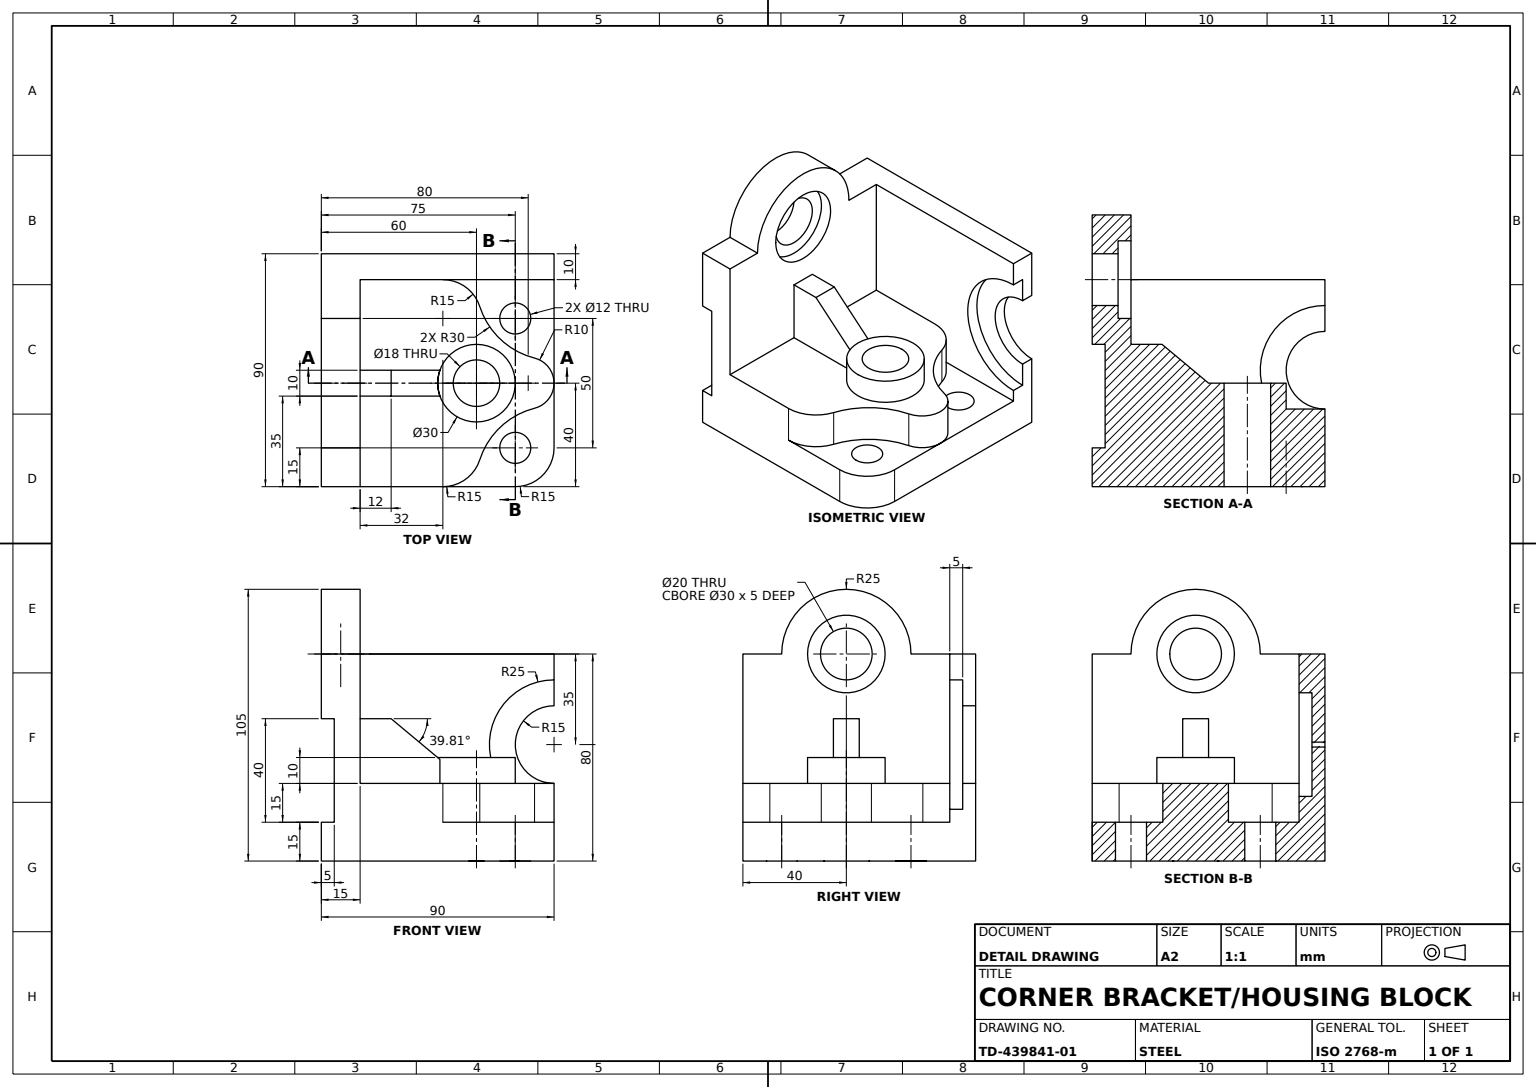
ISO-10303-21;
HEADER;
FILE_DESCRIPTION((''),'2;1');
FILE_NAME('','',(''),(''),'','','');
FILE_SCHEMA(('AUTOMOTIVE_DESIGN'));
ENDSEC;
DATA;
#1=APPLICATION_CONTEXT('');
#2=PRODUCT_CONTEXT('',#1,'mechanical');
#3=PRODUCT('','','',(#2));
#4=PRODUCT_DEFINITION_FORMATION('','',#3);
#5=PRODUCT_DEFINITION_CONTEXT('',#1,'design');
#6=PRODUCT_DEFINITION('','',#4,#5);
#7=PRODUCT_DEFINITION_SHAPE('','',#6);
#8=(LENGTH_UNIT()NAMED_UNIT(*)SI_UNIT(.MILLI.,.METRE.));
#9=(NAMED_UNIT(*)PLANE_ANGLE_UNIT()SI_UNIT($,.RADIAN.));
#10=(NAMED_UNIT(*)SI_UNIT($,.STERADIAN.)SOLID_ANGLE_UNIT());
#11=UNCERTAINTY_MEASURE_WITH_UNIT(LENGTH_MEASURE(1.E-05),#8,'distance_accuracy_value','');
#12=(GEOMETRIC_REPRESENTATION_CONTEXT(3)GLOBAL_UNCERTAINTY_ASSIGNED_CONTEXT((#11))GLOBAL_UNIT_ASSIGNED_CONTEXT((#8,#9,#10))REPRESENTATION_CONTEXT('',''));
#13=CARTESIAN_POINT('',(30.,-0.000006,-19.));
#14=VERTEX_POINT('',#13);
#15=CARTESIAN_POINT('',(30.,15.,-19.));
#16=VERTEX_POINT('',#15);
#17=CARTESIAN_POINT('',(30.,-0.000012,-19.));
#18=DIRECTION('',(0.,1.,0.));
#19=VECTOR('',#18,1000.);
#20=LINE('',#17,#19);
#21=EDGE_CURVE('',#14,#16,#20,.T.);
#22=ORIENTED_EDGE('',*,*,#21,.F.);
#23=CARTESIAN_POINT('',(30.,-0.000006,-31.));
#24=VERTEX_POINT('',#23);
#25=CARTESIAN_POINT('',(29.214602,-0.000012,-19.));
#26=CARTESIAN_POINT('',(28.429513,-0.000012,-19.156164));
#27=CARTESIAN_POINT('',(26.978286,-0.000012,-19.757282));
#28=CARTESIAN_POINT('',(26.31272,-0.000012,-20.201999));
#29=CARTESIAN_POINT('',(25.201999,-0.000012,-21.31272));
#30=CARTESIAN_POINT('',(24.757282,-0.000012,-21.978286));
#31=CARTESIAN_POINT('',(24.156164,-0.000012,-23.429513));
#32=CARTESIAN_POINT('',(24.,-0.000012,-24.214602));
#33=CARTESIAN_POINT('',(24.,-0.000012,-25.785398));
#34=CARTESIAN_POINT('',(24.156164,-0.000012,-26.570487));
#35=CARTESIAN_POINT('',(24.757282,-0.000012,-28.021714));
#36=CARTESIAN_POINT('',(25.201999,-0.000012,-28.68728));
#37=CARTESIAN_POINT('',(26.31272,-0.000012,-29.798001));
#38=CARTESIAN_POINT('',(26.978286,-0.000012,-30.242718));
#39=CARTESIAN_POINT('',(28.429513,-0.000012,-30.843836));
#40=CARTESIAN_POINT('',(29.214602,-0.000012,-31.));
#41=B_SPLINE_CURVE_WITH_KNOTS('',3,(#13,#25,#26,#27,#28,#29,#30,#31,#32,#33,#34,#35,#36,#37,#38,#39,#40,#23),.UNSPECIFIED.,.F.,.F.,(4,2,2,2,2,2,2,2,4),(0.5,0.5625,0.625,0.6875,0.75,0.8125,0.875,0.9375,1.),.UNSPECIFIED.);
#42=EDGE_CURVE('',#14,#24,#41,.T.);
#43=ORIENTED_EDGE('',*,*,#42,.T.);
#44=CARTESIAN_POINT('',(30.,15.,-31.));
#45=VERTEX_POINT('',#44);
#46=CARTESIAN_POINT('',(30.,-0.000012,-31.));
#47=LINE('',#46,#19);
#48=EDGE_CURVE('',#24,#45,#47,.T.);
#49=ORIENTED_EDGE('',*,*,#48,.T.);
#50=CARTESIAN_POINT('',(30.,15.,-25.));
#51=DIRECTION('',(0.,0.,-1.));
#52=AXIS2_PLACEMENT_3D('',#50,#18,#51);
#53=CIRCLE('',#52,6.);
#54=EDGE_CURVE('',#45,#16,#53,.T.);
#55=ORIENTED_EDGE('',*,*,#54,.T.);
#56=EDGE_LOOP('',(#22,#43,#49,#55));
#57=FACE_OUTER_BOUND('',#56,.T.);
#58=CARTESIAN_POINT('',(30.,-0.000012,-25.));
#59=DIRECTION('',(0.,0.,1.));
#60=AXIS2_PLACEMENT_3D('',#58,#18,#59);
#61=CYLINDRICAL_SURFACE('',#60,6.);
#62=ADVANCED_FACE('',(#57),#61,.F.);
#63=CARTESIAN_POINT('',(-45.,80.,-10.));
#64=VERTEX_POINT('',#63);
#65=CARTESIAN_POINT('',(-45.,80.,10.));
#66=VERTEX_POINT('',#65);
#67=CARTESIAN_POINT('',(-45.,80.,0.));
#68=DIRECTION('',(-1.,0.,0.));
#69=AXIS2_PLACEMENT_3D('',#67,#68,#59);
#70=CIRCLE('',#69,10.);
#71=EDGE_CURVE('',#64,#66,#70,.T.);
#72=ORIENTED_EDGE('',*,*,#71,.T.);
#73=CARTESIAN_POINT('',(-35.,80.,10.));
#74=VERTEX_POINT('',#73);
#75=CARTESIAN_POINT('',(-30.,80.,10.));
#76=DIRECTION('',(1.,0.,0.));
#77=VECTOR('',#76,1000.);
#78=LINE('',#75,#77);
#79=EDGE_CURVE('',#66,#74,#78,.T.);
#80=ORIENTED_EDGE('',*,*,#79,.T.);
#81=CARTESIAN_POINT('',(-35.,80.,-10.));
#82=VERTEX_POINT('',#81);
#83=CARTESIAN_POINT('',(-35.,80.,0.));
#84=AXIS2_PLACEMENT_3D('',#83,#76,#51);
#85=CIRCLE('',#84,10.);
#86=EDGE_CURVE('',#74,#82,#85,.T.);
#87=ORIENTED_EDGE('',*,*,#86,.T.);
#88=CARTESIAN_POINT('',(-30.,80.,-10.));
#89=LINE('',#88,#77);
#90=EDGE_CURVE('',#64,#82,#89,.T.);
#91=ORIENTED_EDGE('',*,*,#90,.F.);
#92=EDGE_LOOP('',(#72,#80,#87,#91));
#93=FACE_OUTER_BOUND('',#92,.T.);
#94=CARTESIAN_POINT('',(-30.,80.,0.));
#95=AXIS2_PLACEMENT_3D('',#94,#76,#51);
#96=CYLINDRICAL_SURFACE('',#95,10.);
#97=ADVANCED_FACE('',(#93),#96,.F.);
#98=CARTESIAN_POINT('',(-45.,80.,-25.));
#99=VERTEX_POINT('',#98);
#100=CARTESIAN_POINT('',(-45.,80.,-50.));
#101=VERTEX_POINT('',#100);
#102=CARTESIAN_POINT('',(-45.,80.,-40.));
#103=VECTOR('',#51,1000.);
#104=LINE('',#102,#103);
#105=EDGE_CURVE('',#99,#101,#104,.T.);
#106=ORIENTED_EDGE('',*,*,#105,.F.);
#107=CARTESIAN_POINT('',(-30.,80.,-25.));
#108=VERTEX_POINT('',#107);
#109=VECTOR('',#68,1000.);
#110=LINE('',#107,#109);
#111=EDGE_CURVE('',#108,#99,#110,.T.);
#112=ORIENTED_EDGE('',*,*,#111,.F.);
#113=CARTESIAN_POINT('',(-30.,80.,-40.));
#114=VERTEX_POINT('',#113);
#115=CARTESIAN_POINT('',(-30.,80.,40.));
#116=LINE('',#115,#103);
#117=EDGE_CURVE('',#108,#114,#116,.T.);
#118=ORIENTED_EDGE('',*,*,#117,.T.);
#119=CARTESIAN_POINT('',(45.,80.,-40.));
#120=VERTEX_POINT('',#119);
#121=LINE('',#102,#77);
#122=EDGE_CURVE('',#114,#120,#121,.T.);
#123=ORIENTED_EDGE('',*,*,#122,.T.);
#124=CARTESIAN_POINT('',(45.,80.,-50.));
#125=VERTEX_POINT('',#124);
#126=LINE('',#119,#103);
#127=EDGE_CURVE('',#120,#125,#126,.T.);
#128=ORIENTED_EDGE('',*,*,#127,.T.);
#129=LINE('',#100,#77);
#130=EDGE_CURVE('',#101,#125,#129,.T.);
#131=ORIENTED_EDGE('',*,*,#130,.F.);
#132=EDGE_LOOP('',(#106,#112,#118,#123,#128,#131));
#133=FACE_OUTER_BOUND('',#132,.T.);
#134=AXIS2_PLACEMENT_3D('',#102,#18,#59);
#135=PLANE('',#134);
#136=ADVANCED_FACE('',(#133),#135,.T.);
#137=CARTESIAN_POINT('',(45.,15.,0.));
#138=VERTEX_POINT('',#137);
#139=CARTESIAN_POINT('',(37.460317,15.,-9.692618));
#140=VERTEX_POINT('',#139);
#141=CARTESIAN_POINT('',(35.,15.,0.));
#142=AXIS2_PLACEMENT_3D('',#141,#18,#51);
#143=CIRCLE('',#142,10.);
#144=EDGE_CURVE('',#138,#140,#143,.T.);
#145=ORIENTED_EDGE('',*,*,#144,.T.);
#146=CARTESIAN_POINT('',(37.460317,30.,-9.692618));
#147=VERTEX_POINT('',#146);
#148=DIRECTION('',(0.,-1.,0.));
#149=VECTOR('',#148,1000.);
#150=LINE('',#146,#149);
#151=EDGE_CURVE('',#147,#140,#150,.T.);
#152=ORIENTED_EDGE('',*,*,#151,.F.);
#153=CARTESIAN_POINT('',(37.460317,30.,9.692618));
#154=VERTEX_POINT('',#153);
#155=CARTESIAN_POINT('',(35.,30.,0.));
#156=AXIS2_PLACEMENT_3D('',#155,#18,#59);
#157=CIRCLE('',#156,10.);
#158=EDGE_CURVE('',#154,#147,#157,.T.);
#159=ORIENTED_EDGE('',*,*,#158,.F.);
#160=CARTESIAN_POINT('',(37.460317,15.,9.692618));
#161=VERTEX_POINT('',#160);
#162=LINE('',#153,#149);
#163=EDGE_CURVE('',#154,#161,#162,.T.);
#164=ORIENTED_EDGE('',*,*,#163,.T.);
#165=EDGE_CURVE('',#161,#138,#143,.T.);
#166=ORIENTED_EDGE('',*,*,#165,.T.);
#167=EDGE_LOOP('',(#145,#152,#159,#164,#166));
#168=FACE_OUTER_BOUND('',#167,.T.);
#169=AXIS2_PLACEMENT_3D('',#155,#148,#51);
#170=CYLINDRICAL_SURFACE('',#169,10.);
#171=ADVANCED_FACE('',(#168),#170,.T.);
#172=CARTESIAN_POINT('',(15.,-0.000006,-9.));
#173=VERTEX_POINT('',#172);
#174=CARTESIAN_POINT('',(15.,-0.000006,9.));
#175=VERTEX_POINT('',#174);
#176=CARTESIAN_POINT('',(13.806876,0.,-9.00007));
#177=CARTESIAN_POINT('',(12.658179,0.,-8.77144));
#178=CARTESIAN_POINT('',(10.453519,0.,-7.858391));
#179=CARTESIAN_POINT('',(9.479754,0.,-7.207578));
#180=CARTESIAN_POINT('',(7.792324,0.,-5.520344));
#181=CARTESIAN_POINT('',(7.141737,0.,-4.546427));
#182=CARTESIAN_POINT('',(6.228431,0.,-2.341874));
#183=CARTESIAN_POINT('',(6.00007,0.,-1.193124));
#184=CARTESIAN_POINT('',(5.99993,0.,1.193124));
#185=CARTESIAN_POINT('',(6.22856,0.,2.341821));
#186=CARTESIAN_POINT('',(7.141609,0.,4.546481));
#187=CARTESIAN_POINT('',(7.792422,0.,5.520246));
#188=CARTESIAN_POINT('',(9.479656,0.,7.207676));
#189=CARTESIAN_POINT('',(10.453405,0.,7.858193));
#190=CARTESIAN_POINT('',(12.658294,0.,8.771639));
#191=CARTESIAN_POINT('',(13.806344,0.,9.));
#192=B_SPLINE_CURVE_WITH_KNOTS('',3,(#172,#176,#177,#178,#179,#180,#181,#182,#183,#184,#185,#186,#187,#188,#189,#190,#191,#174),.UNSPECIFIED.,.F.,.F.,(4,2,2,2,2,2,2,2,4),(0.5,0.5625,0.625,0.6875,0.75,0.8125,0.875,0.9375,1.),.UNSPECIFIED.);
#193=EDGE_CURVE('',#173,#175,#192,.T.);
#194=ORIENTED_EDGE('',*,*,#193,.F.);
#195=CARTESIAN_POINT('',(15.,40.,-9.));
#196=VERTEX_POINT('',#195);
#197=LINE('',#195,#149);
#198=EDGE_CURVE('',#196,#173,#197,.T.);
#199=ORIENTED_EDGE('',*,*,#198,.F.);
#200=CARTESIAN_POINT('',(15.,40.,9.));
#201=VERTEX_POINT('',#200);
#202=CARTESIAN_POINT('',(15.,40.,0.));
#203=AXIS2_PLACEMENT_3D('',#202,#18,#59);
#204=CIRCLE('',#203,9.);
#205=EDGE_CURVE('',#196,#201,#204,.T.);
#206=ORIENTED_EDGE('',*,*,#205,.T.);
#207=LINE('',#200,#149);
#208=EDGE_CURVE('',#201,#175,#207,.T.);
#209=ORIENTED_EDGE('',*,*,#208,.T.);
#210=EDGE_LOOP('',(#194,#199,#206,#209));
#211=FACE_OUTER_BOUND('',#210,.T.);
#212=AXIS2_PLACEMENT_3D('',#202,#148,#51);
#213=CYLINDRICAL_SURFACE('',#212,9.);
#214=ADVANCED_FACE('',(#211),#213,.F.);
#215=CARTESIAN_POINT('',(-30.,30.,5.));
#216=VERTEX_POINT('',#215);
#217=CARTESIAN_POINT('',(-30.,55.,5.));
#218=VERTEX_POINT('',#217);
#219=CARTESIAN_POINT('',(-30.,80.,5.));
#220=LINE('',#219,#19);
#221=EDGE_CURVE('',#216,#218,#220,.T.);
#222=ORIENTED_EDGE('',*,*,#221,.F.);
#223=CARTESIAN_POINT('',(0.857864,30.,5.));
#224=VERTEX_POINT('',#223);
#225=CARTESIAN_POINT('',(35.,30.,5.));
#226=LINE('',#225,#77);
#227=EDGE_CURVE('',#216,#224,#226,.T.);
#228=ORIENTED_EDGE('',*,*,#227,.T.);
#229=CARTESIAN_POINT('',(0.857864,39.285113,5.));
#230=VERTEX_POINT('',#229);
#231=CARTESIAN_POINT('',(0.857864,40.,5.));
#232=LINE('',#231,#149);
#233=EDGE_CURVE('',#230,#224,#232,.T.);
#234=ORIENTED_EDGE('',*,*,#233,.F.);
#235=CARTESIAN_POINT('',(-18.,55.,5.));
#236=VERTEX_POINT('',#235);
#237=DIRECTION('',(0.76822128,-0.6401844,0.));
#238=VECTOR('',#237,1000.);
#239=LINE('',#235,#238);
#240=EDGE_CURVE('',#236,#230,#239,.T.);
#241=ORIENTED_EDGE('',*,*,#240,.F.);
#242=CARTESIAN_POINT('',(0.,55.,5.));
#243=LINE('',#242,#77);
#244=EDGE_CURVE('',#218,#236,#243,.T.);
#245=ORIENTED_EDGE('',*,*,#244,.F.);
#246=EDGE_LOOP('',(#222,#228,#234,#241,#245));
#247=FACE_OUTER_BOUND('',#246,.T.);
#248=CARTESIAN_POINT('',(0.,52.388528,5.));
#249=AXIS2_PLACEMENT_3D('',#248,#59,#76);
#250=PLANE('',#249);
#251=ADVANCED_FACE('',(#247),#250,.T.);
#252=CARTESIAN_POINT('',(-40.,55.,-50.));
#253=VERTEX_POINT('',#252);
#254=CARTESIAN_POINT('',(-45.,55.,-50.));
#255=VERTEX_POINT('',#254);
#256=LINE('',#254,#109);
#257=EDGE_CURVE('',#253,#255,#256,.T.);
#258=ORIENTED_EDGE('',*,*,#257,.F.);
#259=CARTESIAN_POINT('',(-40.,55.,40.));
#260=VERTEX_POINT('',#259);
#261=VECTOR('',#59,1000.);
#262=LINE('',#252,#261);
#263=EDGE_CURVE('',#253,#260,#262,.T.);
#264=ORIENTED_EDGE('',*,*,#263,.T.);
#265=CARTESIAN_POINT('',(-45.,55.,40.));
#266=VERTEX_POINT('',#265);
#267=LINE('',#265,#109);
#268=EDGE_CURVE('',#260,#266,#267,.T.);
#269=ORIENTED_EDGE('',*,*,#268,.T.);
#270=LINE('',#254,#261);
#271=EDGE_CURVE('',#255,#266,#270,.T.);
#272=ORIENTED_EDGE('',*,*,#271,.F.);
#273=EDGE_LOOP('',(#258,#264,#269,#272));
#274=FACE_OUTER_BOUND('',#273,.T.);
#275=AXIS2_PLACEMENT_3D('',#254,#18,#59);
#276=PLANE('',#275);
#277=ADVANCED_FACE('',(#274),#276,.F.);
#278=CARTESIAN_POINT('',(2.,30.,-40.));
#279=VERTEX_POINT('',#278);
#280=CARTESIAN_POINT('',(2.,15.,-40.));
#281=VERTEX_POINT('',#280);
#282=LINE('',#278,#149);
#283=EDGE_CURVE('',#279,#281,#282,.T.);
#284=ORIENTED_EDGE('',*,*,#283,.F.);
#285=CARTESIAN_POINT('',(16.280422,30.,-29.590157));
#286=VERTEX_POINT('',#285);
#287=CARTESIAN_POINT('',(2.,30.,-25.));
#288=AXIS2_PLACEMENT_3D('',#287,#148,#51);
#289=CIRCLE('',#288,15.);
#290=EDGE_CURVE('',#279,#286,#289,.T.);
#291=ORIENTED_EDGE('',*,*,#290,.T.);
#292=CARTESIAN_POINT('',(16.280422,15.,-29.590157));
#293=VERTEX_POINT('',#292);
#294=LINE('',#285,#149);
#295=EDGE_CURVE('',#286,#293,#294,.T.);
#296=ORIENTED_EDGE('',*,*,#295,.T.);
#297=CARTESIAN_POINT('',(2.,15.,-25.));
#298=AXIS2_PLACEMENT_3D('',#297,#148,#51);
#299=CIRCLE('',#298,15.);
#300=EDGE_CURVE('',#281,#293,#299,.T.);
#301=ORIENTED_EDGE('',*,*,#300,.F.);
#302=EDGE_LOOP('',(#284,#291,#296,#301));
#303=FACE_OUTER_BOUND('',#302,.T.);
#304=CYLINDRICAL_SURFACE('',#288,15.);
#305=ADVANCED_FACE('',(#303),#304,.T.);
#306=CARTESIAN_POINT('',(15.,40.,-15.));
#307=VERTEX_POINT('',#306);
#308=CARTESIAN_POINT('',(0.,40.,0.));
#309=VERTEX_POINT('',#308);
#310=CIRCLE('',#203,15.);
#311=EDGE_CURVE('',#307,#309,#310,.T.);
#312=ORIENTED_EDGE('',*,*,#311,.F.);
#313=CARTESIAN_POINT('',(15.,30.,-15.));
#314=VERTEX_POINT('',#313);
#315=LINE('',#306,#149);
#316=EDGE_CURVE('',#307,#314,#315,.T.);
#317=ORIENTED_EDGE('',*,*,#316,.T.);
#318=CARTESIAN_POINT('',(0.857864,30.,-5.));
#319=VERTEX_POINT('',#318);
#320=CARTESIAN_POINT('',(15.,30.,0.));
#321=AXIS2_PLACEMENT_3D('',#320,#148,#59);
#322=CIRCLE('',#321,15.);
#323=EDGE_CURVE('',#319,#314,#322,.T.);
#324=ORIENTED_EDGE('',*,*,#323,.F.);
#325=CARTESIAN_POINT('',(0.857864,39.285113,-5.));
#326=VERTEX_POINT('',#325);
#327=CARTESIAN_POINT('',(0.857864,40.,-5.));
#328=LINE('',#327,#149);
#329=EDGE_CURVE('',#326,#319,#328,.T.);
#330=ORIENTED_EDGE('',*,*,#329,.F.);
#331=CARTESIAN_POINT('',(0.288727,39.759394,-3.390236));
#332=CARTESIAN_POINT('',(0.,40.,-1.707413));
#333=(BOUNDED_CURVE()B_SPLINE_CURVE(3,(#325,#331,#332,#308),.UNSPECIFIED.,.F.,.F.)B_SPLINE_CURVE_WITH_KNOTS((4,4),(2.801755744,3.141592654),.UNSPECIFIED.)CURVE()GEOMETRIC_REPRESENTATION_ITEM()RATIONAL_B_SPLINE_CURVE((1.,0.99039904,0.99039904,1.))REPRESENTATION_ITEM(''));
#334=EDGE_CURVE('',#326,#309,#333,.T.);
#335=ORIENTED_EDGE('',*,*,#334,.T.);
#336=EDGE_LOOP('',(#312,#317,#324,#330,#335));
#337=FACE_OUTER_BOUND('',#336,.T.);
#338=CYLINDRICAL_SURFACE('',#212,15.);
#339=ADVANCED_FACE('',(#337),#338,.T.);
#340=ORIENTED_EDGE('',*,*,#122,.F.);
#341=CARTESIAN_POINT('',(-30.,30.,-40.));
#342=VERTEX_POINT('',#341);
#343=CARTESIAN_POINT('',(-30.,15.,-40.));
#344=LINE('',#343,#149);
#345=EDGE_CURVE('',#114,#342,#344,.T.);
#346=ORIENTED_EDGE('',*,*,#345,.T.);
#347=LINE('',#341,#77);
#348=EDGE_CURVE('',#342,#279,#347,.T.);
#349=ORIENTED_EDGE('',*,*,#348,.T.);
#350=ORIENTED_EDGE('',*,*,#283,.T.);
#351=CARTESIAN_POINT('',(45.,15.,-40.));
#352=VERTEX_POINT('',#351);
#353=CARTESIAN_POINT('',(-45.,15.,-40.));
#354=LINE('',#353,#109);
#355=EDGE_CURVE('',#352,#281,#354,.T.);
#356=ORIENTED_EDGE('',*,*,#355,.F.);
#357=CARTESIAN_POINT('',(45.,20.,-40.));
#358=VERTEX_POINT('',#357);
#359=LINE('',#351,#149);
#360=EDGE_CURVE('',#358,#352,#359,.T.);
#361=ORIENTED_EDGE('',*,*,#360,.F.);
#362=CARTESIAN_POINT('',(45.,70.,-40.));
#363=VERTEX_POINT('',#362);
#364=CARTESIAN_POINT('',(45.,45.,-40.));
#365=AXIS2_PLACEMENT_3D('',#364,#59,#76);
#366=CIRCLE('',#365,25.);
#367=EDGE_CURVE('',#363,#358,#366,.T.);
#368=ORIENTED_EDGE('',*,*,#367,.F.);
#369=EDGE_CURVE('',#120,#363,#359,.T.);
#370=ORIENTED_EDGE('',*,*,#369,.F.);
#371=EDGE_LOOP('',(#340,#346,#349,#350,#356,#361,#368,#370));
#372=FACE_OUTER_BOUND('',#371,.T.);
#373=CARTESIAN_POINT('',(0.,0.,-40.));
#374=AXIS2_PLACEMENT_3D('',#373,#51,#68);
#375=PLANE('',#374);
#376=ADVANCED_FACE('',(#372),#375,.F.);
#377=CARTESIAN_POINT('',(-30.,55.,-5.));
#378=VERTEX_POINT('',#377);
#379=CARTESIAN_POINT('',(-30.,55.,0.));
#380=LINE('',#379,#103);
#381=EDGE_CURVE('',#218,#378,#380,.T.);
#382=ORIENTED_EDGE('',*,*,#381,.F.);
#383=ORIENTED_EDGE('',*,*,#244,.T.);
#384=CARTESIAN_POINT('',(-18.,55.,-5.));
#385=VERTEX_POINT('',#384);
#386=CARTESIAN_POINT('',(-18.,55.,0.));
#387=LINE('',#386,#261);
#388=EDGE_CURVE('',#385,#236,#387,.T.);
#389=ORIENTED_EDGE('',*,*,#388,.F.);
#390=CARTESIAN_POINT('',(0.,55.,-5.));
#391=LINE('',#390,#77);
#392=EDGE_CURVE('',#378,#385,#391,.T.);
#393=ORIENTED_EDGE('',*,*,#392,.F.);
#394=EDGE_LOOP('',(#382,#383,#389,#393));
#395=FACE_OUTER_BOUND('',#394,.T.);
#396=AXIS2_PLACEMENT_3D('',#379,#148,#76);
#397=PLANE('',#396);
#398=ADVANCED_FACE('',(#395),#397,.F.);
#399=CARTESIAN_POINT('',(2.,15.,40.));
#400=VERTEX_POINT('',#399);
#401=CARTESIAN_POINT('',(16.280422,15.,29.590157));
#402=VERTEX_POINT('',#401);
#403=CARTESIAN_POINT('',(2.,15.,25.));
#404=AXIS2_PLACEMENT_3D('',#403,#18,#51);
#405=CIRCLE('',#404,15.);
#406=EDGE_CURVE('',#400,#402,#405,.T.);
#407=ORIENTED_EDGE('',*,*,#406,.T.);
#408=CARTESIAN_POINT('',(16.280422,30.,29.590157));
#409=VERTEX_POINT('',#408);
#410=LINE('',#408,#149);
#411=EDGE_CURVE('',#409,#402,#410,.T.);
#412=ORIENTED_EDGE('',*,*,#411,.F.);
#413=CARTESIAN_POINT('',(2.,30.,40.));
#414=VERTEX_POINT('',#413);
#415=CARTESIAN_POINT('',(2.,30.,25.));
#416=AXIS2_PLACEMENT_3D('',#415,#18,#59);
#417=CIRCLE('',#416,15.);
#418=EDGE_CURVE('',#414,#409,#417,.T.);
#419=ORIENTED_EDGE('',*,*,#418,.F.);
#420=LINE('',#413,#149);
#421=EDGE_CURVE('',#414,#400,#420,.T.);
#422=ORIENTED_EDGE('',*,*,#421,.T.);
#423=EDGE_LOOP('',(#407,#412,#419,#422));
#424=FACE_OUTER_BOUND('',#423,.T.);
#425=AXIS2_PLACEMENT_3D('',#415,#148,#51);
#426=CYLINDRICAL_SURFACE('',#425,15.);
#427=ADVANCED_FACE('',(#424),#426,.T.);
#428=CARTESIAN_POINT('',(-40.,15.,-50.));
#429=VERTEX_POINT('',#428);
#430=CARTESIAN_POINT('',(-40.,15.,40.));
#431=VERTEX_POINT('',#430);
#432=LINE('',#428,#261);
#433=EDGE_CURVE('',#429,#431,#432,.T.);
#434=ORIENTED_EDGE('',*,*,#433,.F.);
#435=CARTESIAN_POINT('',(-45.,15.,-50.));
#436=VERTEX_POINT('',#435);
#437=LINE('',#435,#77);
#438=EDGE_CURVE('',#436,#429,#437,.T.);
#439=ORIENTED_EDGE('',*,*,#438,.F.);
#440=CARTESIAN_POINT('',(-45.,15.,40.));
#441=VERTEX_POINT('',#440);
#442=LINE('',#435,#261);
#443=EDGE_CURVE('',#436,#441,#442,.T.);
#444=ORIENTED_EDGE('',*,*,#443,.T.);
#445=LINE('',#440,#77);
#446=EDGE_CURVE('',#441,#431,#445,.T.);
#447=ORIENTED_EDGE('',*,*,#446,.T.);
#448=EDGE_LOOP('',(#434,#439,#444,#447));
#449=FACE_OUTER_BOUND('',#448,.T.);
#450=AXIS2_PLACEMENT_3D('',#435,#148,#76);
#451=PLANE('',#450);
#452=ADVANCED_FACE('',(#449),#451,.F.);
#453=ORIENTED_EDGE('',*,*,#369,.T.);
#454=CARTESIAN_POINT('',(45.,70.,-45.));
#455=VERTEX_POINT('',#454);
#456=LINE('',#454,#261);
#457=EDGE_CURVE('',#455,#363,#456,.T.);
#458=ORIENTED_EDGE('',*,*,#457,.F.);
#459=CARTESIAN_POINT('',(45.,60.,-45.));
#460=VERTEX_POINT('',#459);
#461=CARTESIAN_POINT('',(45.,0.,-45.));
#462=LINE('',#461,#19);
#463=EDGE_CURVE('',#460,#455,#462,.T.);
#464=ORIENTED_EDGE('',*,*,#463,.F.);
#465=CARTESIAN_POINT('',(45.,60.,-50.));
#466=VERTEX_POINT('',#465);
#467=CARTESIAN_POINT('',(45.,60.,-50.001));
#468=LINE('',#467,#261);
#469=EDGE_CURVE('',#466,#460,#468,.T.);
#470=ORIENTED_EDGE('',*,*,#469,.F.);
#471=CARTESIAN_POINT('',(45.,15.,-50.));
#472=LINE('',#471,#149);
#473=EDGE_CURVE('',#125,#466,#472,.T.);
#474=ORIENTED_EDGE('',*,*,#473,.F.);
#475=ORIENTED_EDGE('',*,*,#127,.F.);
#476=EDGE_LOOP('',(#453,#458,#464,#470,#474,#475));
#477=FACE_OUTER_BOUND('',#476,.T.);
#478=AXIS2_PLACEMENT_3D('',#471,#76,#51);
#479=PLANE('',#478);
#480=ADVANCED_FACE('',(#477),#479,.T.);
#481=CARTESIAN_POINT('',(0.,40.,1.707413));
#482=CARTESIAN_POINT('',(0.288727,39.759394,3.390236));
#483=(BOUNDED_CURVE()B_SPLINE_CURVE(3,(#308,#481,#482,#229),.UNSPECIFIED.,.F.,.F.)B_SPLINE_CURVE_WITH_KNOTS((4,4),(3.141592654,3.481429563),.UNSPECIFIED.)CURVE()GEOMETRIC_REPRESENTATION_ITEM()RATIONAL_B_SPLINE_CURVE((1.,0.99039904,0.99039904,1.))REPRESENTATION_ITEM(''));
#484=EDGE_CURVE('',#309,#230,#483,.T.);
#485=ORIENTED_EDGE('',*,*,#484,.T.);
#486=ORIENTED_EDGE('',*,*,#233,.T.);
#487=CARTESIAN_POINT('',(15.,30.,15.));
#488=VERTEX_POINT('',#487);
#489=EDGE_CURVE('',#488,#224,#322,.T.);
#490=ORIENTED_EDGE('',*,*,#489,.F.);
#491=CARTESIAN_POINT('',(15.,40.,15.));
#492=VERTEX_POINT('',#491);
#493=LINE('',#491,#149);
#494=EDGE_CURVE('',#492,#488,#493,.T.);
#495=ORIENTED_EDGE('',*,*,#494,.F.);
#496=EDGE_CURVE('',#309,#492,#310,.T.);
#497=ORIENTED_EDGE('',*,*,#496,.F.);
#498=EDGE_LOOP('',(#485,#486,#490,#495,#497));
#499=FACE_OUTER_BOUND('',#498,.T.);
#500=ADVANCED_FACE('',(#499),#338,.T.);
#501=ORIENTED_EDGE('',*,*,#130,.T.);
#502=ORIENTED_EDGE('',*,*,#473,.T.);
#503=CARTESIAN_POINT('',(45.,30.,-50.));
#504=VERTEX_POINT('',#503);
#505=CARTESIAN_POINT('',(45.,45.,-50.));
#506=AXIS2_PLACEMENT_3D('',#505,#59,#68);
#507=CIRCLE('',#506,15.);
#508=EDGE_CURVE('',#466,#504,#507,.T.);
#509=ORIENTED_EDGE('',*,*,#508,.T.);
#510=CARTESIAN_POINT('',(45.,0.,-50.));
#511=VERTEX_POINT('',#510);
#512=EDGE_CURVE('',#504,#511,#472,.T.);
#513=ORIENTED_EDGE('',*,*,#512,.T.);
#514=CARTESIAN_POINT('',(-45.,0.,-50.));
#515=VERTEX_POINT('',#514);
#516=LINE('',#514,#77);
#517=EDGE_CURVE('',#515,#511,#516,.T.);
#518=ORIENTED_EDGE('',*,*,#517,.F.);
#519=LINE('',#435,#149);
#520=EDGE_CURVE('',#436,#515,#519,.T.);
#521=ORIENTED_EDGE('',*,*,#520,.F.);
#522=ORIENTED_EDGE('',*,*,#438,.T.);
#523=LINE('',#252,#19);
#524=EDGE_CURVE('',#429,#253,#523,.T.);
#525=ORIENTED_EDGE('',*,*,#524,.T.);
#526=ORIENTED_EDGE('',*,*,#257,.T.);
#527=EDGE_CURVE('',#101,#255,#519,.T.);
#528=ORIENTED_EDGE('',*,*,#527,.F.);
#529=EDGE_LOOP('',(#501,#502,#509,#513,#518,#521,#522,#525,#526,#528));
#530=FACE_OUTER_BOUND('',#529,.T.);
#531=AXIS2_PLACEMENT_3D('',#435,#51,#68);
#532=PLANE('',#531);
#533=ADVANCED_FACE('',(#530),#532,.T.);
#534=ORIENTED_EDGE('',*,*,#311,.T.);
#535=ORIENTED_EDGE('',*,*,#496,.T.);
#536=EDGE_CURVE('',#492,#307,#310,.T.);
#537=ORIENTED_EDGE('',*,*,#536,.T.);
#538=EDGE_LOOP('',(#534,#535,#537));
#539=FACE_OUTER_BOUND('',#538,.T.);
#540=EDGE_CURVE('',#201,#196,#204,.T.);
#541=ORIENTED_EDGE('',*,*,#540,.F.);
#542=ORIENTED_EDGE('',*,*,#205,.F.);
#543=EDGE_LOOP('',(#541,#542));
#544=FACE_BOUND('',#543,.T.);
#545=PLANE('',#203);
#546=ADVANCED_FACE('',(#539,#544),#545,.T.);
#547=ORIENTED_EDGE('',*,*,#208,.F.);
#548=ORIENTED_EDGE('',*,*,#540,.T.);
#549=ORIENTED_EDGE('',*,*,#198,.T.);
#550=CARTESIAN_POINT('',(16.193292,0.,9.));
#551=CARTESIAN_POINT('',(17.341821,0.,8.77144));
#552=CARTESIAN_POINT('',(19.546481,0.,7.858391));
#553=CARTESIAN_POINT('',(20.520246,0.,7.207578));
#554=CARTESIAN_POINT('',(22.207676,0.,5.520344));
#555=CARTESIAN_POINT('',(22.858263,0.,4.546427));
#556=CARTESIAN_POINT('',(23.771569,0.,2.341874));
#557=CARTESIAN_POINT('',(23.99993,0.,1.193124));
#558=CARTESIAN_POINT('',(24.00007,0.,-1.193124));
#559=CARTESIAN_POINT('',(23.77144,0.,-2.341821));
#560=CARTESIAN_POINT('',(22.858391,0.,-4.546481));
#561=CARTESIAN_POINT('',(22.207578,0.,-5.520246));
#562=CARTESIAN_POINT('',(20.520344,0.,-7.207676));
#563=CARTESIAN_POINT('',(19.546427,0.,-7.858263));
#564=CARTESIAN_POINT('',(17.341874,0.,-8.771569));
#565=CARTESIAN_POINT('',(16.193124,0.,-8.99993));
#566=B_SPLINE_CURVE_WITH_KNOTS('',3,(#174,#550,#551,#552,#553,#554,#555,#556,#557,#558,#559,#560,#561,#562,#563,#564,#565,#172),.UNSPECIFIED.,.F.,.F.,(4,2,2,2,2,2,2,2,4),(0.,0.0625,0.125,0.1875,0.25,0.3125,0.375,0.4375,0.5),.UNSPECIFIED.);
#567=EDGE_CURVE('',#175,#173,#566,.T.);
#568=ORIENTED_EDGE('',*,*,#567,.F.);
#569=EDGE_LOOP('',(#547,#548,#549,#568));
#570=FACE_OUTER_BOUND('',#569,.T.);
#571=ADVANCED_FACE('',(#570),#213,.F.);
#572=CARTESIAN_POINT('',(30.,15.,31.));
#573=VERTEX_POINT('',#572);
#574=CARTESIAN_POINT('',(30.,15.,19.));
#575=VERTEX_POINT('',#574);
#576=CARTESIAN_POINT('',(30.,15.,25.));
#577=AXIS2_PLACEMENT_3D('',#576,#148,#51);
#578=CIRCLE('',#577,6.);
#579=EDGE_CURVE('',#573,#575,#578,.T.);
#580=ORIENTED_EDGE('',*,*,#579,.F.);
#581=CARTESIAN_POINT('',(30.,-0.000006,31.));
#582=VERTEX_POINT('',#581);
#583=CARTESIAN_POINT('',(30.,-0.000012,31.));
#584=LINE('',#583,#19);
#585=EDGE_CURVE('',#582,#573,#584,.T.);
#586=ORIENTED_EDGE('',*,*,#585,.F.);
#587=CARTESIAN_POINT('',(30.,-0.000006,19.));
#588=VERTEX_POINT('',#587);
#589=CARTESIAN_POINT('',(29.204701,0.,18.99993));
#590=CARTESIAN_POINT('',(28.438687,0.,19.152439));
#591=CARTESIAN_POINT('',(26.969112,0.,19.761006));
#592=CARTESIAN_POINT('',(26.31977,0.,20.195047));
#593=CARTESIAN_POINT('',(25.194948,0.,21.319672));
#594=CARTESIAN_POINT('',(24.761135,0.,21.969165));
#595=CARTESIAN_POINT('',(24.152311,0.,23.438634));
#596=CARTESIAN_POINT('',(24.00007,0.,24.204701));
#597=CARTESIAN_POINT('',(23.99993,0.,25.795299));
#598=CARTESIAN_POINT('',(24.152439,0.,26.561313));
#599=CARTESIAN_POINT('',(24.761006,0.,28.030888));
#600=CARTESIAN_POINT('',(25.195047,0.,28.68023));
#601=CARTESIAN_POINT('',(26.319672,0.,29.805052));
#602=CARTESIAN_POINT('',(26.968997,0.,30.238795));
#603=CARTESIAN_POINT('',(28.438802,0.,30.847759));
#604=CARTESIAN_POINT('',(29.204169,0.,31.));
#605=B_SPLINE_CURVE_WITH_KNOTS('',3,(#587,#589,#590,#591,#592,#593,#594,#595,#596,#597,#598,#599,#600,#601,#602,#603,#604,#581),.UNSPECIFIED.,.F.,.F.,(4,2,2,2,2,2,2,2,4),(0.5,0.5625,0.625,0.6875,0.75,0.8125,0.875,0.9375,1.),.UNSPECIFIED.);
#606=EDGE_CURVE('',#588,#582,#605,.T.);
#607=ORIENTED_EDGE('',*,*,#606,.F.);
#608=CARTESIAN_POINT('',(30.,-0.000012,19.));
#609=LINE('',#608,#19);
#610=EDGE_CURVE('',#588,#575,#609,.T.);
#611=ORIENTED_EDGE('',*,*,#610,.T.);
#612=EDGE_LOOP('',(#580,#586,#607,#611));
#613=FACE_OUTER_BOUND('',#612,.T.);
#614=CARTESIAN_POINT('',(30.,-0.000012,25.));
#615=AXIS2_PLACEMENT_3D('',#614,#18,#59);
#616=CYLINDRICAL_SURFACE('',#615,6.);
#617=ADVANCED_FACE('',(#613),#616,.F.);
#618=CARTESIAN_POINT('',(44.841266,30.,38.770472));
#619=AXIS2_PLACEMENT_3D('',#618,#18,#59);
#620=CIRCLE('',#619,30.);
#621=EDGE_CURVE('',#154,#409,#620,.T.);
#622=ORIENTED_EDGE('',*,*,#621,.T.);
#623=ORIENTED_EDGE('',*,*,#411,.T.);
#624=CARTESIAN_POINT('',(44.841266,15.,38.770472));
#625=AXIS2_PLACEMENT_3D('',#624,#18,#51);
#626=CIRCLE('',#625,30.);
#627=EDGE_CURVE('',#161,#402,#626,.T.);
#628=ORIENTED_EDGE('',*,*,#627,.F.);
#629=ORIENTED_EDGE('',*,*,#163,.F.);
#630=EDGE_LOOP('',(#622,#623,#628,#629));
#631=FACE_OUTER_BOUND('',#630,.T.);
#632=AXIS2_PLACEMENT_3D('',#618,#148,#51);
#633=CYLINDRICAL_SURFACE('',#632,30.);
#634=ADVANCED_FACE('',(#631),#633,.F.);
#635=ORIENTED_EDGE('',*,*,#367,.T.);
#636=CARTESIAN_POINT('',(45.,20.,-45.));
#637=VERTEX_POINT('',#636);
#638=LINE('',#636,#261);
#639=EDGE_CURVE('',#637,#358,#638,.T.);
#640=ORIENTED_EDGE('',*,*,#639,.F.);
#641=CARTESIAN_POINT('',(45.,45.,-45.));
#642=AXIS2_PLACEMENT_3D('',#641,#59,#76);
#643=CIRCLE('',#642,25.);
#644=EDGE_CURVE('',#455,#637,#643,.T.);
#645=ORIENTED_EDGE('',*,*,#644,.F.);
#646=ORIENTED_EDGE('',*,*,#457,.T.);
#647=EDGE_LOOP('',(#635,#640,#645,#646));
#648=FACE_OUTER_BOUND('',#647,.T.);
#649=CYLINDRICAL_SURFACE('',#642,25.);
#650=ADVANCED_FACE('',(#648),#649,.F.);
#651=CARTESIAN_POINT('',(-30.,80.,25.));
#652=VERTEX_POINT('',#651);
#653=CARTESIAN_POINT('',(-45.,80.,25.));
#654=VERTEX_POINT('',#653);
#655=LINE('',#651,#109);
#656=EDGE_CURVE('',#652,#654,#655,.T.);
#657=ORIENTED_EDGE('',*,*,#656,.T.);
#658=CARTESIAN_POINT('',(-45.,80.,40.));
#659=VERTEX_POINT('',#658);
#660=LINE('',#658,#103);
#661=EDGE_CURVE('',#659,#654,#660,.T.);
#662=ORIENTED_EDGE('',*,*,#661,.F.);
#663=VERTEX_POINT('',#115);
#664=LINE('',#115,#109);
#665=EDGE_CURVE('',#663,#659,#664,.T.);
#666=ORIENTED_EDGE('',*,*,#665,.F.);
#667=EDGE_CURVE('',#663,#652,#116,.T.);
#668=ORIENTED_EDGE('',*,*,#667,.T.);
#669=EDGE_LOOP('',(#657,#662,#666,#668));
#670=FACE_OUTER_BOUND('',#669,.T.);
#671=AXIS2_PLACEMENT_3D('',#115,#18,#59);
#672=PLANE('',#671);
#673=ADVANCED_FACE('',(#670),#672,.T.);
#674=LINE('',#259,#19);
#675=EDGE_CURVE('',#431,#260,#674,.T.);
#676=ORIENTED_EDGE('',*,*,#675,.T.);
#677=ORIENTED_EDGE('',*,*,#263,.F.);
#678=ORIENTED_EDGE('',*,*,#524,.F.);
#679=ORIENTED_EDGE('',*,*,#433,.T.);
#680=EDGE_LOOP('',(#676,#677,#678,#679));
#681=FACE_OUTER_BOUND('',#680,.T.);
#682=AXIS2_PLACEMENT_3D('',#252,#76,#18);
#683=PLANE('',#682);
#684=ADVANCED_FACE('',(#681),#683,.F.);
#685=ORIENTED_EDGE('',*,*,#86,.F.);
#686=EDGE_CURVE('',#82,#74,#85,.T.);
#687=ORIENTED_EDGE('',*,*,#686,.F.);
#688=EDGE_LOOP('',(#685,#687));
#689=FACE_BOUND('',#688,.T.);
#690=CARTESIAN_POINT('',(-35.,80.,15.));
#691=VERTEX_POINT('',#690);
#692=CARTESIAN_POINT('',(-35.,80.,-15.));
#693=VERTEX_POINT('',#692);
#694=CIRCLE('',#84,15.);
#695=EDGE_CURVE('',#691,#693,#694,.T.);
#696=ORIENTED_EDGE('',*,*,#695,.T.);
#697=EDGE_CURVE('',#693,#691,#694,.T.);
#698=ORIENTED_EDGE('',*,*,#697,.T.);
#699=EDGE_LOOP('',(#696,#698));
#700=FACE_OUTER_BOUND('',#699,.T.);
#701=CARTESIAN_POINT('',(-35.,90.,0.));
#702=AXIS2_PLACEMENT_3D('',#701,#68,#59);
#703=PLANE('',#702);
#704=ADVANCED_FACE('',(#689,#700),#703,.F.);
#705=CARTESIAN_POINT('',(45.,0.,25.));
#706=VERTEX_POINT('',#705);
#707=LINE('',#510,#261);
#708=EDGE_CURVE('',#511,#706,#707,.T.);
#709=ORIENTED_EDGE('',*,*,#708,.T.);
#710=CARTESIAN_POINT('',(30.,0.,40.));
#711=VERTEX_POINT('',#710);
#712=CARTESIAN_POINT('',(30.,0.,25.));
#713=AXIS2_PLACEMENT_3D('',#712,#148,#51);
#714=CIRCLE('',#713,15.);
#715=EDGE_CURVE('',#706,#711,#714,.T.);
#716=ORIENTED_EDGE('',*,*,#715,.T.);
#717=CARTESIAN_POINT('',(-45.,0.,40.));
#718=VERTEX_POINT('',#717);
#719=CARTESIAN_POINT('',(45.,0.,40.));
#720=LINE('',#719,#109);
#721=EDGE_CURVE('',#711,#718,#720,.T.);
#722=ORIENTED_EDGE('',*,*,#721,.T.);
#723=LINE('',#717,#103);
#724=EDGE_CURVE('',#718,#515,#723,.T.);
#725=ORIENTED_EDGE('',*,*,#724,.T.);
#726=ORIENTED_EDGE('',*,*,#517,.T.);
#727=EDGE_LOOP('',(#709,#716,#722,#725,#726));
#728=FACE_OUTER_BOUND('',#727,.T.);
#729=ORIENTED_EDGE('',*,*,#606,.T.);
#730=CARTESIAN_POINT('',(30.795468,0.,31.));
#731=CARTESIAN_POINT('',(31.561313,0.,30.847561));
#732=CARTESIAN_POINT('',(33.030888,0.,30.238994));
#733=CARTESIAN_POINT('',(33.68023,0.,29.804953));
#734=CARTESIAN_POINT('',(34.805052,0.,28.680328));
#735=CARTESIAN_POINT('',(35.238865,0.,28.030835));
#736=CARTESIAN_POINT('',(35.847689,0.,26.561366));
#737=CARTESIAN_POINT('',(35.99993,0.,25.795299));
#738=CARTESIAN_POINT('',(36.00007,0.,24.204701));
#739=CARTESIAN_POINT('',(35.847561,0.,23.438687));
#740=CARTESIAN_POINT('',(35.238994,0.,21.969112));
#741=CARTESIAN_POINT('',(34.804953,0.,21.31977));
#742=CARTESIAN_POINT('',(33.680328,0.,20.194948));
#743=CARTESIAN_POINT('',(33.030835,0.,19.761135));
#744=CARTESIAN_POINT('',(31.561366,0.,19.152311));
#745=CARTESIAN_POINT('',(30.795299,0.,19.00007));
#746=B_SPLINE_CURVE_WITH_KNOTS('',3,(#581,#730,#731,#732,#733,#734,#735,#736,#737,#738,#739,#740,#741,#742,#743,#744,#745,#587),.UNSPECIFIED.,.F.,.F.,(4,2,2,2,2,2,2,2,4),(0.,0.0625,0.125,0.1875,0.25,0.3125,0.375,0.4375,0.5),.UNSPECIFIED.);
#747=EDGE_CURVE('',#582,#588,#746,.T.);
#748=ORIENTED_EDGE('',*,*,#747,.T.);
#749=EDGE_LOOP('',(#729,#748));
#750=FACE_BOUND('',#749,.T.);
#751=CARTESIAN_POINT('',(30.785398,-0.000012,-31.));
#752=CARTESIAN_POINT('',(31.570487,-0.000012,-30.843836));
#753=CARTESIAN_POINT('',(33.021714,-0.000012,-30.242718));
#754=CARTESIAN_POINT('',(33.68728,-0.000012,-29.798001));
#755=CARTESIAN_POINT('',(34.798001,-0.000012,-28.68728));
#756=CARTESIAN_POINT('',(35.242718,-0.000012,-28.021714));
#757=CARTESIAN_POINT('',(35.843836,-0.000012,-26.570487));
#758=CARTESIAN_POINT('',(36.,-0.000012,-25.785398));
#759=CARTESIAN_POINT('',(36.,-0.000012,-24.214602));
#760=CARTESIAN_POINT('',(35.843836,-0.000012,-23.429513));
#761=CARTESIAN_POINT('',(35.242718,-0.000012,-21.978286));
#762=CARTESIAN_POINT('',(34.798001,-0.000012,-21.31272));
#763=CARTESIAN_POINT('',(33.68728,-0.000012,-20.201999));
#764=CARTESIAN_POINT('',(33.021714,-0.000012,-19.757282));
#765=CARTESIAN_POINT('',(31.570487,-0.000012,-19.156164));
#766=CARTESIAN_POINT('',(30.785398,-0.000012,-19.));
#767=B_SPLINE_CURVE_WITH_KNOTS('',3,(#23,#751,#752,#753,#754,#755,#756,#757,#758,#759,#760,#761,#762,#763,#764,#765,#766,#13),.UNSPECIFIED.,.F.,.F.,(4,2,2,2,2,2,2,2,4),(0.,0.0625,0.125,0.1875,0.25,0.3125,0.375,0.4375,0.5),.UNSPECIFIED.);
#768=EDGE_CURVE('',#24,#14,#767,.T.);
#769=ORIENTED_EDGE('',*,*,#768,.F.);
#770=ORIENTED_EDGE('',*,*,#42,.F.);
#771=EDGE_LOOP('',(#769,#770));
#772=FACE_BOUND('',#771,.T.);
#773=ORIENTED_EDGE('',*,*,#567,.T.);
#774=ORIENTED_EDGE('',*,*,#193,.T.);
#775=EDGE_LOOP('',(#773,#774));
#776=FACE_BOUND('',#775,.T.);
#777=CARTESIAN_POINT('',(0.,0.,0.));
#778=AXIS2_PLACEMENT_3D('',#777,#148,#51);
#779=PLANE('',#778);
#780=ADVANCED_FACE('',(#728,#750,#772,#776),#779,.T.);
#781=ORIENTED_EDGE('',*,*,#334,.F.);
#782=LINE('',#384,#238);
#783=EDGE_CURVE('',#385,#326,#782,.T.);
#784=ORIENTED_EDGE('',*,*,#783,.F.);
#785=ORIENTED_EDGE('',*,*,#388,.T.);
#786=ORIENTED_EDGE('',*,*,#240,.T.);
#787=ORIENTED_EDGE('',*,*,#484,.F.);
#788=EDGE_LOOP('',(#781,#784,#785,#786,#787));
#789=FACE_OUTER_BOUND('',#788,.T.);
#790=DIRECTION('',(-0.6401844,-0.76822128,0.));
#791=AXIS2_PLACEMENT_3D('',#386,#790,#237);
#792=PLANE('',#791);
#793=ADVANCED_FACE('',(#789),#792,.F.);
#794=ORIENTED_EDGE('',*,*,#54,.F.);
#795=EDGE_CURVE('',#16,#45,#53,.T.);
#796=ORIENTED_EDGE('',*,*,#795,.F.);
#797=EDGE_LOOP('',(#794,#796));
#798=FACE_BOUND('',#797,.T.);
#799=ORIENTED_EDGE('',*,*,#144,.F.);
#800=LINE('',#471,#261);
#801=EDGE_CURVE('',#352,#138,#800,.T.);
#802=ORIENTED_EDGE('',*,*,#801,.F.);
#803=ORIENTED_EDGE('',*,*,#355,.T.);
#804=ORIENTED_EDGE('',*,*,#300,.T.);
#805=CARTESIAN_POINT('',(44.841266,15.,-38.770472));
#806=AXIS2_PLACEMENT_3D('',#805,#148,#51);
#807=CIRCLE('',#806,30.);
#808=EDGE_CURVE('',#140,#293,#807,.T.);
#809=ORIENTED_EDGE('',*,*,#808,.F.);
#810=EDGE_LOOP('',(#799,#802,#803,#804,#809));
#811=FACE_OUTER_BOUND('',#810,.T.);
#812=CARTESIAN_POINT('',(0.,15.,0.));
#813=AXIS2_PLACEMENT_3D('',#812,#148,#51);
#814=PLANE('',#813);
#815=ADVANCED_FACE('',(#798,#811),#814,.F.);
#816=ORIENTED_EDGE('',*,*,#329,.T.);
#817=CARTESIAN_POINT('',(-30.,30.,-5.));
#818=VERTEX_POINT('',#817);
#819=CARTESIAN_POINT('',(35.,30.,-5.));
#820=LINE('',#819,#77);
#821=EDGE_CURVE('',#818,#319,#820,.T.);
#822=ORIENTED_EDGE('',*,*,#821,.F.);
#823=CARTESIAN_POINT('',(-30.,80.,-5.));
#824=LINE('',#823,#19);
#825=EDGE_CURVE('',#818,#378,#824,.T.);
#826=ORIENTED_EDGE('',*,*,#825,.T.);
#827=ORIENTED_EDGE('',*,*,#392,.T.);
#828=ORIENTED_EDGE('',*,*,#783,.T.);
#829=EDGE_LOOP('',(#816,#822,#826,#827,#828));
#830=FACE_OUTER_BOUND('',#829,.T.);
#831=CARTESIAN_POINT('',(0.,52.388528,-5.));
#832=AXIS2_PLACEMENT_3D('',#831,#59,#76);
#833=PLANE('',#832);
#834=ADVANCED_FACE('',(#830),#833,.F.);
#835=ORIENTED_EDGE('',*,*,#111,.T.);
#836=CIRCLE('',#69,25.);
#837=EDGE_CURVE('',#654,#99,#836,.T.);
#838=ORIENTED_EDGE('',*,*,#837,.F.);
#839=ORIENTED_EDGE('',*,*,#656,.F.);
#840=AXIS2_PLACEMENT_3D('',#94,#68,#59);
#841=CIRCLE('',#840,25.);
#842=EDGE_CURVE('',#652,#108,#841,.T.);
#843=ORIENTED_EDGE('',*,*,#842,.T.);
#844=EDGE_LOOP('',(#835,#838,#839,#843));
#845=FACE_OUTER_BOUND('',#844,.T.);
#846=CYLINDRICAL_SURFACE('',#840,25.);
#847=ADVANCED_FACE('',(#845),#846,.T.);
#848=CARTESIAN_POINT('',(45.,30.,-45.));
#849=VERTEX_POINT('',#848);
#850=CIRCLE('',#642,15.);
#851=EDGE_CURVE('',#460,#849,#850,.T.);
#852=ORIENTED_EDGE('',*,*,#851,.F.);
#853=ORIENTED_EDGE('',*,*,#463,.T.);
#854=ORIENTED_EDGE('',*,*,#644,.T.);
#855=EDGE_CURVE('',#637,#849,#462,.T.);
#856=ORIENTED_EDGE('',*,*,#855,.T.);
#857=EDGE_LOOP('',(#852,#853,#854,#856));
#858=FACE_OUTER_BOUND('',#857,.T.);
#859=CARTESIAN_POINT('',(0.,0.,-45.));
#860=AXIS2_PLACEMENT_3D('',#859,#59,#76);
#861=PLANE('',#860);
#862=ADVANCED_FACE('',(#858),#861,.T.);
#863=ORIENTED_EDGE('',*,*,#536,.F.);
#864=ORIENTED_EDGE('',*,*,#494,.T.);
#865=EDGE_CURVE('',#314,#488,#322,.T.);
#866=ORIENTED_EDGE('',*,*,#865,.F.);
#867=ORIENTED_EDGE('',*,*,#316,.F.);
#868=EDGE_LOOP('',(#863,#864,#866,#867));
#869=FACE_OUTER_BOUND('',#868,.T.);
#870=ADVANCED_FACE('',(#869),#338,.T.);
#871=ORIENTED_EDGE('',*,*,#579,.T.);
#872=EDGE_CURVE('',#575,#573,#578,.T.);
#873=ORIENTED_EDGE('',*,*,#872,.T.);
#874=EDGE_LOOP('',(#871,#873));
#875=FACE_BOUND('',#874,.T.);
#876=ORIENTED_EDGE('',*,*,#165,.F.);
#877=ORIENTED_EDGE('',*,*,#627,.T.);
#878=ORIENTED_EDGE('',*,*,#406,.F.);
#879=CARTESIAN_POINT('',(30.,15.,40.));
#880=VERTEX_POINT('',#879);
#881=CARTESIAN_POINT('',(45.,15.,40.));
#882=LINE('',#881,#109);
#883=EDGE_CURVE('',#880,#400,#882,.T.);
#884=ORIENTED_EDGE('',*,*,#883,.F.);
#885=CARTESIAN_POINT('',(45.,15.,25.));
#886=VERTEX_POINT('',#885);
#887=AXIS2_PLACEMENT_3D('',#576,#18,#51);
#888=CIRCLE('',#887,15.);
#889=EDGE_CURVE('',#880,#886,#888,.T.);
#890=ORIENTED_EDGE('',*,*,#889,.T.);
#891=EDGE_CURVE('',#138,#886,#800,.T.);
#892=ORIENTED_EDGE('',*,*,#891,.F.);
#893=EDGE_LOOP('',(#876,#877,#878,#884,#890,#892));
#894=FACE_OUTER_BOUND('',#893,.T.);
#895=ADVANCED_FACE('',(#875,#894),#814,.F.);
#896=ORIENTED_EDGE('',*,*,#610,.F.);
#897=ORIENTED_EDGE('',*,*,#747,.F.);
#898=ORIENTED_EDGE('',*,*,#585,.T.);
#899=ORIENTED_EDGE('',*,*,#872,.F.);
#900=EDGE_LOOP('',(#896,#897,#898,#899));
#901=FACE_OUTER_BOUND('',#900,.T.);
#902=ADVANCED_FACE('',(#901),#616,.F.);
#903=ORIENTED_EDGE('',*,*,#855,.F.);
#904=ORIENTED_EDGE('',*,*,#639,.T.);
#905=ORIENTED_EDGE('',*,*,#360,.T.);
#906=ORIENTED_EDGE('',*,*,#801,.T.);
#907=ORIENTED_EDGE('',*,*,#891,.T.);
#908=LINE('',#885,#149);
#909=EDGE_CURVE('',#886,#706,#908,.T.);
#910=ORIENTED_EDGE('',*,*,#909,.T.);
#911=ORIENTED_EDGE('',*,*,#708,.F.);
#912=ORIENTED_EDGE('',*,*,#512,.F.);
#913=CARTESIAN_POINT('',(45.,30.,-50.001));
#914=LINE('',#913,#261);
#915=EDGE_CURVE('',#504,#849,#914,.T.);
#916=ORIENTED_EDGE('',*,*,#915,.T.);
#917=EDGE_LOOP('',(#903,#904,#905,#906,#907,#910,#911,#912,#916));
#918=FACE_OUTER_BOUND('',#917,.T.);
#919=ADVANCED_FACE('',(#918),#479,.T.);
#920=ORIENTED_EDGE('',*,*,#915,.F.);
#921=ORIENTED_EDGE('',*,*,#508,.F.);
#922=ORIENTED_EDGE('',*,*,#469,.T.);
#923=ORIENTED_EDGE('',*,*,#851,.T.);
#924=EDGE_LOOP('',(#920,#921,#922,#923));
#925=FACE_OUTER_BOUND('',#924,.T.);
#926=CARTESIAN_POINT('',(45.,45.,-50.001));
#927=AXIS2_PLACEMENT_3D('',#926,#59,#76);
#928=CYLINDRICAL_SURFACE('',#927,15.);
#929=ADVANCED_FACE('',(#925),#928,.F.);
#930=EDGE_CURVE('',#66,#64,#70,.T.);
#931=ORIENTED_EDGE('',*,*,#930,.F.);
#932=ORIENTED_EDGE('',*,*,#71,.F.);
#933=EDGE_LOOP('',(#931,#932));
#934=FACE_BOUND('',#933,.T.);
#935=ORIENTED_EDGE('',*,*,#271,.T.);
#936=LINE('',#440,#149);
#937=EDGE_CURVE('',#659,#266,#936,.T.);
#938=ORIENTED_EDGE('',*,*,#937,.F.);
#939=ORIENTED_EDGE('',*,*,#661,.T.);
#940=ORIENTED_EDGE('',*,*,#837,.T.);
#941=ORIENTED_EDGE('',*,*,#105,.T.);
#942=ORIENTED_EDGE('',*,*,#527,.T.);
#943=EDGE_LOOP('',(#935,#938,#939,#940,#941,#942));
#944=FACE_OUTER_BOUND('',#943,.T.);
#945=AXIS2_PLACEMENT_3D('',#440,#68,#59);
#946=PLANE('',#945);
#947=ADVANCED_FACE('',(#934,#944),#946,.T.);
#948=ORIENTED_EDGE('',*,*,#715,.F.);
#949=ORIENTED_EDGE('',*,*,#909,.F.);
#950=ORIENTED_EDGE('',*,*,#889,.F.);
#951=LINE('',#879,#19);
#952=EDGE_CURVE('',#711,#880,#951,.T.);
#953=ORIENTED_EDGE('',*,*,#952,.F.);
#954=EDGE_LOOP('',(#948,#949,#950,#953));
#955=FACE_OUTER_BOUND('',#954,.T.);
#956=CYLINDRICAL_SURFACE('',#577,15.);
#957=ADVANCED_FACE('',(#955),#956,.T.);
#958=ORIENTED_EDGE('',*,*,#795,.T.);
#959=ORIENTED_EDGE('',*,*,#48,.F.);
#960=ORIENTED_EDGE('',*,*,#768,.T.);
#961=ORIENTED_EDGE('',*,*,#21,.T.);
#962=EDGE_LOOP('',(#958,#959,#960,#961));
#963=FACE_OUTER_BOUND('',#962,.T.);
#964=ADVANCED_FACE('',(#963),#61,.F.);
#965=CARTESIAN_POINT('',(44.841266,30.,-38.770472));
#966=AXIS2_PLACEMENT_3D('',#965,#148,#51);
#967=CIRCLE('',#966,30.);
#968=EDGE_CURVE('',#147,#286,#967,.T.);
#969=ORIENTED_EDGE('',*,*,#968,.F.);
#970=ORIENTED_EDGE('',*,*,#151,.T.);
#971=ORIENTED_EDGE('',*,*,#808,.T.);
#972=ORIENTED_EDGE('',*,*,#295,.F.);
#973=EDGE_LOOP('',(#969,#970,#971,#972));
#974=FACE_OUTER_BOUND('',#973,.T.);
#975=CYLINDRICAL_SURFACE('',#966,30.);
#976=ADVANCED_FACE('',(#974),#975,.F.);
#977=ORIENTED_EDGE('',*,*,#520,.T.);
#978=ORIENTED_EDGE('',*,*,#724,.F.);
#979=EDGE_CURVE('',#441,#718,#936,.T.);
#980=ORIENTED_EDGE('',*,*,#979,.F.);
#981=ORIENTED_EDGE('',*,*,#443,.F.);
#982=EDGE_LOOP('',(#977,#978,#980,#981));
#983=FACE_OUTER_BOUND('',#982,.T.);
#984=ADVANCED_FACE('',(#983),#946,.T.);
#985=ORIENTED_EDGE('',*,*,#268,.F.);
#986=ORIENTED_EDGE('',*,*,#675,.F.);
#987=ORIENTED_EDGE('',*,*,#446,.F.);
#988=ORIENTED_EDGE('',*,*,#979,.T.);
#989=ORIENTED_EDGE('',*,*,#721,.F.);
#990=ORIENTED_EDGE('',*,*,#952,.T.);
#991=ORIENTED_EDGE('',*,*,#883,.T.);
#992=ORIENTED_EDGE('',*,*,#421,.F.);
#993=CARTESIAN_POINT('',(-30.,30.,40.));
#994=VERTEX_POINT('',#993);
#995=LINE('',#993,#77);
#996=EDGE_CURVE('',#994,#414,#995,.T.);
#997=ORIENTED_EDGE('',*,*,#996,.F.);
#998=CARTESIAN_POINT('',(-30.,15.,40.));
#999=LINE('',#998,#19);
#1000=EDGE_CURVE('',#994,#663,#999,.T.);
#1001=ORIENTED_EDGE('',*,*,#1000,.T.);
#1002=ORIENTED_EDGE('',*,*,#665,.T.);
#1003=ORIENTED_EDGE('',*,*,#937,.T.);
#1004=EDGE_LOOP('',(#985,#986,#987,#988,#989,#990,#991,#992,#997,#1001,#1002,#1003));
#1005=FACE_OUTER_BOUND('',#1004,.T.);
#1006=AXIS2_PLACEMENT_3D('',#881,#59,#76);
#1007=PLANE('',#1006);
#1008=ADVANCED_FACE('',(#1005),#1007,.T.);
#1009=CARTESIAN_POINT('',(-30.,80.,-15.));
#1010=VERTEX_POINT('',#1009);
#1011=LINE('',#1009,#77);
#1012=EDGE_CURVE('',#693,#1010,#1011,.T.);
#1013=ORIENTED_EDGE('',*,*,#1012,.T.);
#1014=CARTESIAN_POINT('',(-30.,80.,15.));
#1015=VERTEX_POINT('',#1014);
#1016=CIRCLE('',#95,15.);
#1017=EDGE_CURVE('',#1010,#1015,#1016,.T.);
#1018=ORIENTED_EDGE('',*,*,#1017,.T.);
#1019=LINE('',#1014,#77);
#1020=EDGE_CURVE('',#691,#1015,#1019,.T.);
#1021=ORIENTED_EDGE('',*,*,#1020,.F.);
#1022=ORIENTED_EDGE('',*,*,#697,.F.);
#1023=EDGE_LOOP('',(#1013,#1018,#1021,#1022));
#1024=FACE_OUTER_BOUND('',#1023,.T.);
#1025=CYLINDRICAL_SURFACE('',#95,15.);
#1026=ADVANCED_FACE('',(#1024),#1025,.F.);
#1027=EDGE_CURVE('',#1015,#1010,#1016,.T.);
#1028=ORIENTED_EDGE('',*,*,#1027,.T.);
#1029=ORIENTED_EDGE('',*,*,#1012,.F.);
#1030=ORIENTED_EDGE('',*,*,#695,.F.);
#1031=ORIENTED_EDGE('',*,*,#1020,.T.);
#1032=EDGE_LOOP('',(#1028,#1029,#1030,#1031));
#1033=FACE_OUTER_BOUND('',#1032,.T.);
#1034=ADVANCED_FACE('',(#1033),#1025,.F.);
#1035=ORIENTED_EDGE('',*,*,#79,.F.);
#1036=ORIENTED_EDGE('',*,*,#930,.T.);
#1037=ORIENTED_EDGE('',*,*,#90,.T.);
#1038=ORIENTED_EDGE('',*,*,#686,.T.);
#1039=EDGE_LOOP('',(#1035,#1036,#1037,#1038));
#1040=FACE_OUTER_BOUND('',#1039,.T.);
#1041=ADVANCED_FACE('',(#1040),#96,.F.);
#1042=ORIENTED_EDGE('',*,*,#323,.T.);
#1043=ORIENTED_EDGE('',*,*,#865,.T.);
#1044=ORIENTED_EDGE('',*,*,#489,.T.);
#1045=ORIENTED_EDGE('',*,*,#227,.F.);
#1046=LINE('',#993,#103);
#1047=EDGE_CURVE('',#994,#216,#1046,.T.);
#1048=ORIENTED_EDGE('',*,*,#1047,.F.);
#1049=ORIENTED_EDGE('',*,*,#996,.T.);
#1050=ORIENTED_EDGE('',*,*,#418,.T.);
#1051=ORIENTED_EDGE('',*,*,#621,.F.);
#1052=ORIENTED_EDGE('',*,*,#158,.T.);
#1053=ORIENTED_EDGE('',*,*,#968,.T.);
#1054=ORIENTED_EDGE('',*,*,#290,.F.);
#1055=ORIENTED_EDGE('',*,*,#348,.F.);
#1056=EDGE_CURVE('',#818,#342,#1046,.T.);
#1057=ORIENTED_EDGE('',*,*,#1056,.F.);
#1058=ORIENTED_EDGE('',*,*,#821,.T.);
#1059=EDGE_LOOP('',(#1042,#1043,#1044,#1045,#1048,#1049,#1050,#1051,#1052,#1053,#1054,#1055,#1057,#1058));
#1060=FACE_OUTER_BOUND('',#1059,.T.);
#1061=PLANE('',#156);
#1062=ADVANCED_FACE('',(#1060),#1061,.T.);
#1063=ORIENTED_EDGE('',*,*,#1027,.F.);
#1064=ORIENTED_EDGE('',*,*,#1017,.F.);
#1065=EDGE_LOOP('',(#1063,#1064));
#1066=FACE_BOUND('',#1065,.T.);
#1067=ORIENTED_EDGE('',*,*,#825,.F.);
#1068=ORIENTED_EDGE('',*,*,#1056,.T.);
#1069=ORIENTED_EDGE('',*,*,#345,.F.);
#1070=ORIENTED_EDGE('',*,*,#117,.F.);
#1071=ORIENTED_EDGE('',*,*,#842,.F.);
#1072=ORIENTED_EDGE('',*,*,#667,.F.);
#1073=ORIENTED_EDGE('',*,*,#1000,.F.);
#1074=ORIENTED_EDGE('',*,*,#1047,.T.);
#1075=ORIENTED_EDGE('',*,*,#221,.T.);
#1076=ORIENTED_EDGE('',*,*,#381,.T.);
#1077=EDGE_LOOP('',(#1067,#1068,#1069,#1070,#1071,#1072,#1073,#1074,#1075,#1076));
#1078=FACE_OUTER_BOUND('',#1077,.T.);
#1079=PLANE('',#840);
#1080=ADVANCED_FACE('',(#1066,#1078),#1079,.F.);
#1081=CLOSED_SHELL('',(#62,#97,#136,#171,#214,#251,#277,#305,#339,#376,#398,#427,#452,#480,#500,#533,#546,#571,#617,#634,#650,#673,#684,#704,#780,#793,#815,#834,#847,#862,#870,#895,#902,#919,#929,#947,#957,#964,#976,#984,#1008,#1026,#1034,#1041,#1062,#1080));
#1082=MANIFOLD_SOLID_BREP('',#1081);
#1083=ADVANCED_BREP_SHAPE_REPRESENTATION('',(#1082),#12);
#1084=SHAPE_DEFINITION_REPRESENTATION(#7,#1083);
ENDSEC;
END-ISO-10303-21;
